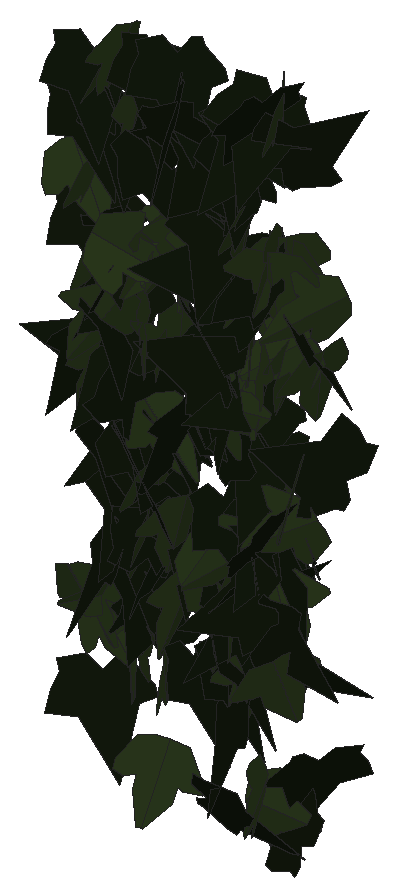
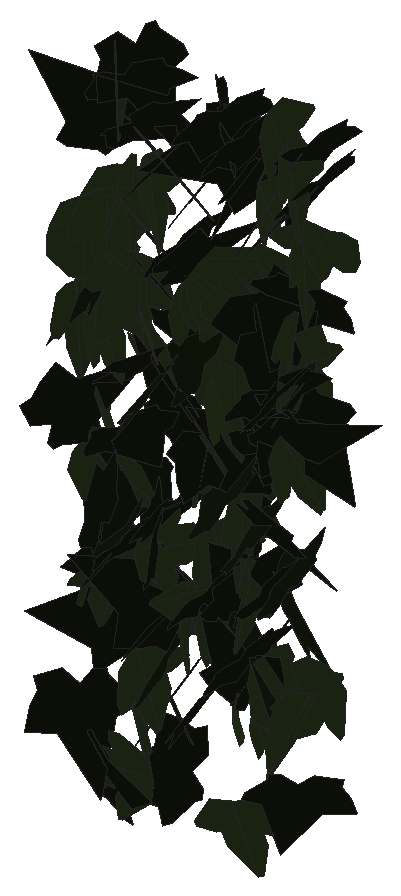
# SketchUp Ruby script. Lengths in inches.
U = 1.inch
M = Sketchup.active_model
def pt(a) = Geom::Point3d.new(a.map { |v| v * U })
def face(e, loops, mat)
  f = e.add_face(loops[0].map { |a| pt(a) })
  loops[1..].each { |l| e.add_face(l.map { |a| pt(a) }).erase! }
  f.material = f.back_material = mat if mat
  f
end
# faces: each face lists its corners as indices into pts; further lists are holes
def faces(e, pts, list, mat = nil) = list.each { |f| face(e, (f[0].is_a?(Array) ? f : [f]).map { |l| l.map { |i| pts[i] } }, mat) }
# xy, xz, yz: faces in a plane at the given z, y or x. An outline is a flat list of corners, or four numbers for a rectangle; further outlines are holes
def ring(l) = l.size == 4 ? [[l[0], l[1]], [l[2], l[1]], [l[2], l[3]], [l[0], l[3]]] : l.each_slice(2).to_a
def flat(e, list, mat, &to3) = list.each { |f| face(e, (f[0].is_a?(Array) ? f : [f]).map { |l| ring(l).map { |u, v| to3.(u, v) } }, mat) }
def xy(e, z, list, mat = nil) = flat(e, list, mat) { |x, y| [x, y, z] }
def xz(e, y, list, mat = nil) = flat(e, list, mat) { |x, z| [x, y, z] }
def yz(e, x, list, mat = nil) = flat(e, list, mat) { |y, z| [x, y, z] }
def lines(e, pts, list) = list.each { |a, b| e.add_line(pt(pts[a]), pt(pts[b])) }
# prism: a flat outline (further loops are holes) pulled along v
def prism(e, loops, v, mat = nil)
  f = face(e, loops, mat); d = Geom::Vector3d.new(v.map { |x| x * U })
  f.pushpull(f.normal.samedirection?(d) ? d.length : -d.length)
end
def box(e, o, s, mat = nil) = prism(e, [[o, [o[0] + s[0], o[1], o[2]], [o[0] + s[0], o[1] + s[1], o[2]], [o[0], o[1] + s[1], o[2]]]], [0, 0, s[2]], mat)
def at(x, y, z, deg = 0) = Geom::Transformation.translation(pt([x, y, z])) * Geom::Transformation.rotation(ORIGIN, Z_AXIS, deg.degrees)
def axes(o, x, y, z) = Geom::Transformation.new([*x, 0, *y, 0, *z, 0, *pt(o).to_a, 1])
def part(name) = M.definitions.add(name)
# library, detail: a bought-in or finely detailed component or shape, given as its bounding box
def library(name, o, s) = part(name).tap { |d| box(d.entities, o, s) }
def detail(e, o, s) = box(e.add_group.entities, o, s)
def put(e, d, t, mat = nil) = e.add_instance(d, t).tap { |i| i.material = mat if mat }
def group(e, t, mat = nil) = e.add_group.tap { |g| g.transformation = t; g.material = mat if mat }.entities
root = M.entities
M.materials.add("efeu1").color = [18, 25, 13]
M.materials.add("efeu2").color = [43, 57, 29]
c1 = part("ivyleaf_9")
p = [[1.54,2.16,1.25],[1.36,2.04,1.19],[-0.21,0.99,0.68],[-0.71,1.11,0.82],[-0.85,0.86,0.67],[-0.8,0.17,0.21],
  [-0.9,-0.01,0.1],[-0.67,-0.16,-0.02],[-0.08,-0.08,-0.05],[-0.03,-0.6,-0.4],[0.65,-0.88,-0.66],[0.83,-0.6,-0.49],
  [1.29,-0.42,-0.43],[1.8125,-0.07,-0.26],[1.21,0.44,0.15]]
faces(c1.entities,p,[[0,1,2,3,4,5,6,7,8,9,10,11,12,13,14]],"efeu1")
c2 = part("ivyleaf_10")
p = [[0,0.5,-0.03],[-0.0625,2.02,-0.43],[-0.19,2.01,-0.46],[-0.54,1.05,-0.29],[-0.52,0.625,-0.18],[-0.83,0.76,-0.28],
  [-1.16,0.64,-0.33],[-1.15,0.33,-0.24],[-0.77,-0.39,0.02],[-0.3,-0.51,0.16],[0.04,-0.48,0.23],[-0.02,2.01,-0.4375],
  [-0.06,2.01,-0.43],[0.04,-0.49,0.23],[0.67,-0.49,0.14],[1.38,0.36,-0.2],[1.375,0.51,-0.24],[0.81,0.65,-0.19],
  [0.62,0.59,-0.15],[0.6,1.09,-0.28],[0.5,1.23,-0.31]]
faces(c2.entities,p,[[0,1,2,3,4,5,6,7,8,9,10],[11,12,0,13,14,15,16,17,18,19,20]],"efeu2")
put(root,c1,axes([31.45,222.08,226.97],[0.14956,-0.33063,0.34397],[-0.15429,0.30759,0.36275],[-0.45147,-0.21465,-0.01002]))
put(root,c2,axes([30.55,222.25,229.83],[-0.21795,-0.34953,0.28342],[-0.15304,-0.23856,-0.4119],[0.42317,-0.2663,-0.00299]))
put(root,c2,axes([33.16,222.05,223.6],[0.30428,-0.36826,-0.14765],[-0.08218,0.12353,-0.47748],[0.38815,0.31484,0.01465]))
put(root,c1,axes([30.61,222.21,226.32],[-0.40272,0.13792,-0.26228],[0.23987,-0.10813,-0.42517],[-0.174,-0.46828,0.02093]))
put(root,c1,axes([31.2,222.05,232.53],[0.22113,-0.38594,-0.22837],[-0.10686,0.20194,-0.44475],[0.43552,0.2455,0.00682]))
put(root,c2,axes([33.5,221.99,225.47],[-0.27696,-0.38547,-0.15717],[0.0796,0.13626,-0.47444],[0.4086,-0.28783,-0.01411]))
put(root,c1,axes([32.36,222.05,223.1],[0.41261,-0.11866,0.25626],[0.24759,-0.06623,-0.42932],[0.13583,0.48118,0.0041]))
put(root,c1,axes([31.6,222.28,233.29],[-0.27418,0.11213,-0.4028],[0.37252,-0.15324,-0.29623],[-0.18989,-0.46254,0.00049]))
put(root,c1,axes([32.27,222.45,230.77],[-0.2241,-0.0434,0.44485],[-0.31262,-0.34045,-0.1907],[0.31945,-0.36361,0.12545]))
put(root,c1,axes([32.58,222.27,224.45],[-0.35983,0.05267,-0.34314],[0.33766,-0.06174,-0.36356],[-0.08067,-0.49337,0.00886]))
put(root,c1,axes([33.2,222.12,226],[0.04453,-0.04723,-0.49577],[0.44248,0.23216,0.01763],[0.22853,-0.44031,0.06247]))
put(root,c1,axes([33.13,222.16,226.34],[-0.44882,0.14556,0.16544],[-0.15751,0.0506,-0.47184],[-0.15411,-0.47566,0.00043]))
put(root,c2,axes([33.35,222.09,231.46],[-0.4619,-0.19142,0.00291],[-0.00274,-0.00098,-0.49999],[0.19142,-0.46191,-0.00014]))
put(root,c2,axes([33.2,222.41,231.48],[-0.02504,0.27389,-0.41756],[0.01105,-0.41768,-0.27463],[-0.49925,-0.02298,0.01487]))
put(root,c2,axes([32.4,222.28,228.9375],[0.08497,-0.1088,-0.48056],[0.42623,-0.22842,0.12708],[-0.24719,-0.43126,0.05394]))
put(root,c2,axes([30.66,222,230.87],[0.15039,0.11673,0.46234],[0.379,0.26494,-0.19017],[-0.28938,0.40766,-0.00879]))
put(root,c1,axes([30.03,222.28,232.76],[0.13252,-0.47272,-0.09475],[0.0012,0.09859,-0.49018],[0.48212,0.12969,0.02727]))
put(root,c1,axes([32.46,222.14,229.5],[-0.27431,0.13469,0.39574],[-0.35996,0.16457,-0.30552],[-0.21256,-0.45252,0.00668]))
put(root,c1,axes([33.19,222.24,231.21],[-0.45908,0.1956,0.03148],[-0.02973,0.01054,-0.499],[-0.19587,-0.46003,0.00195]))
put(root,c1,axes([32.82,222.29,226.01],[-0.46992,0.15477,-0.07226],[0.06609,-0.03029,-0.49469],[-0.1575,-0.47448,0.00801]))
put(root,c1,axes([32.34,222.21,228.26],[-0.20283,0.17516,0.42211],[0.29655,-0.30094,0.26738],[0.34773,0.35882,0.01819]))
put(root,c2,axes([31.2,222.49,224.57],[-0.00541,0.02291,0.49945],[0.40198,-0.2968,0.01797],[0.29729,0.40173,-0.01521]))
put(root,c2,axes([31.6,222.45,225.875],[0.02998,-0.44579,0.22443],[0.05607,-0.2204,-0.44528],[0.49594,0.05187,0.03677]))
put(root,c1,axes([33.21,221.85,227.34],[0.10913,0.42255,0.24402],[0.06265,0.23584,-0.43641],[-0.48391,0.12583,-0.00147]))
put(root,c1,axes([30.0625,222.44,233.33],[-0.02975,-0.49473,-0.06601],[0.01847,0.065,-0.49541],[0.49877,-0.03191,0.01441]))
put(root,c1,axes([33.04,222.25,233.67],[-0.06447,0.41498,-0.27135],[0.03559,-0.26906,-0.41993],[-0.49455,-0.07346,0.00515]))
put(root,c2,axes([32.45,222.63,226.62],[-0.00025,-0.09169,0.49152],[-0.02745,-0.49078,-0.09157],[0.49925,-0.02703,-0.00479]))
put(root,c2,axes([32.75,222.39,229.68],[0.41358,-0.14747,0.23918],[0.22269,-0.08751,-0.43903],[0.17135,0.46967,-0.0067]))
put(root,c1,axes([30.79,222.63,225.39],[0.01053,-0.37536,0.33014],[0.02863,-0.32922,-0.37523],[0.49907,0.0268,0.01456]))
put(root,c1,axes([30.29,222.55,229.55],[0.12032,-0.43719,0.21068],[0.06195,-0.20145,-0.45341],[0.48134,0.13521,0.00569]))
put(root,c1,axes([30.26,222.39,229.23],[0.02593,0.28829,-0.40769],[-0.01629,-0.40754,-0.28922],[-0.49906,0.02828,-0.01174]))
put(root,c2,axes([30.79,222.53,229.62],[-0.15141,0.16736,-0.44617],[0.2085,-0.39769,-0.21993],[-0.42849,-0.25265,0.05064]))
put(root,c2,axes([33.87,222.61,230.84],[-0.0705,-0.18459,0.4593],[-0.16812,-0.42743,-0.19758],[0.46558,-0.18229,-0.0018]))
put(root,c2,axes([33.46,222.42,228.25],[0.31377,-0.37857,0.0907],[0.05557,-0.07174,-0.4917],[0.3853,0.31864,-0.00294]))
put(root,c2,axes([33.59,222.43,227.5],[-0.22618,-0.11469,0.43092],[-0.36823,-0.22448,-0.25302],[0.25151,-0.4318,0.01708]))
put(root,c2,axes([29.97,222.23,231.87],[0.37134,0.27532,0.19055],[0.15152,0.11557,-0.46226],[-0.29858,0.40105,0.0024]))
put(root,c1,axes([31.72,222.49,228.49],[-0.10576,0.25807,-0.41499],[0.12603,-0.39583,-0.27827],[-0.47216,-0.16346,0.01867]))
put(root,c2,axes([32.36,222.31,225.8],[0.38459,-0.30392,-0.0986],[-0.04094,0.10615,-0.48688],[0.31688,0.38258,0.05677]))
put(root,c2,axes([31.21,222.35,228.36],[-0.39728,-0.12288,-0.27761],[0.30065,-0.09576,-0.38786],[0.04216,-0.47511,0.14998]))
put(root,c1,axes([33,222.69,229.1],[-0.35126,-0.14312,0.32577],[-0.18958,-0.31212,-0.34153],[0.30112,-0.36346,0.165]))
put(root,c2,axes([32.72,222.34,231.95],[0.11405,-0.47814,-0.09149],[-0.01916,0.08949,-0.49155],[0.48644,0.11563,0.00209]))
put(root,c1,axes([30.14,222.45,231.15],[-0.21262,-0.28904,-0.34821],[0.29254,0.20574,-0.34941],[0.34527,-0.35231,0.08163]))
put(root,c1,axes([31.74,222.76,232.1],[-0.10251,-0.31373,0.37559],[-0.00552,-0.38298,-0.3214],[0.48935,-0.07004,0.07506]))
put(root,c1,axes([32,222.69,231.32],[-0.07971,-0.47321,0.14042],[0.0014,-0.14246,-0.47927],[0.4936,-0.07601,0.02403]))
put(root,c1,axes([32.88,222.28,232.4],[-0.35996,0.28801,0.19359],[-0.16122,0.10821,-0.46076],[-0.3073,-0.39413,0.01497]))
put(root,c1,axes([31.31,222.1,232.77],[0.0628,0.1577,-0.47031],[0.20494,0.42346,0.16936],[0.45173,-0.21404,-0.01145]))
put(root,c1,axes([32.9,222.625,233.47],[-0.29716,-0.39646,-0.06717],[0.03296,0.05923,-0.49538],[0.40076,-0.29884,-0.00906]))
put(root,c2,axes([30.15,222.37,231.75],[0.06623,-0.48218,-0.11454],[0.01015,0.11686,-0.48605],[0.49549,0.06206,0.02527]))
put(root,c1,axes([30.82,222.19,228.27],[-0.03168,-0.05473,0.49599],[0.47762,0.14058,0.04602],[-0.14449,0.4767,0.04337]))
put(root,c2,axes([33.4375,222.53,230.1],[-0.30616,0.01098,0.39515],[-0.35543,-0.22639,-0.2691],[0.17301,-0.44568,0.14642]))
put(root,c1,axes([30.55,222.79,226.68],[-0.10428,-0.42688,0.23853],[-0.03437,-0.23689,-0.43898],[0.48779,-0.10795,0.02006]))
put(root,c1,axes([32.67,222.77,232.92],[-0.29058,-0.37259,0.16354],[-0.06611,-0.15506,-0.47073],[0.40149,-0.29519,0.04085]))
put(root,c2,axes([31.5,222.5,226.99],[-0.07434,-0.49198,0.04925],[-0.00015,-0.04978,-0.49752],[0.49444,-0.07398,0.00725]))
put(root,c1,axes([32.29,222.75,232.42],[0.01345,-0.46907,0.1726],[0.04795,-0.17065,-0.46752],[0.49751,0.02913,0.04039]))
put(root,c2,axes([30.18,222.63,228.86],[-0.00834,-0.46213,0.19071],[-0.01572,-0.1904,-0.46206],[0.49968,-0.01371,-0.01135]))
put(root,c2,axes([29.87,222.41,225.39],[-0.44855,0.07356,-0.2083],[0.20392,-0.04343,-0.45446],[-0.08495,-0.49265,0.00896]))
put(root,c2,axes([32.87,222.5,223.0625],[-0.0275,0.0027,-0.49924],[0.47636,-0.14949,-0.02705],[-0.14941,-0.47712,0.00565]))
put(root,c1,axes([30.6,222.73,229.05],[-0.38326,-0.31425,0.06602],[-0.04363,-0.05088,-0.49549],[0.31813,-0.38556,0.01157]))
put(root,c2,axes([30.48,222.74,224.45],[-0.10948,0.1082,-0.47572],[0.20763,-0.43086,-0.14578],[-0.44148,-0.22947,0.04941]))
put(root,c2,axes([31.42,222.51,229.28],[-0.48567,-0.07669,0.09078],[0.0906,0.00822,0.49166],[-0.0769,0.49401,0.00591]))
put(root,c1,axes([30.42,222.71,228.82],[-0.25914,-0.27677,-0.32595],[-0.10576,-0.32781,0.36243],[-0.41432,0.25679,0.11135]))
put(root,c2,axes([30.4,222.64,233.57],[0.05833,-0.46831,0.16518],[0.04309,-0.16092,-0.47143],[0.49471,0.06923,0.02158]))
put(root,c1,axes([32.22,222.5,227.33],[0.14804,-0.43981,-0.18615],[-0.05579,0.17763,-0.46404],[0.47431,0.15816,0.00352]))
put(root,c1,axes([32.78,222.49,230.62],[-0.44872,0.20334,0.08543],[-0.08032,0.02972,-0.49261],[-0.20541,-0.45582,0.006]))
put(root,c1,axes([30.65,222.7,230.46],[-0.24181,0.17685,-0.40032],[0.2012,-0.36123,-0.28112],[-0.38865,-0.29704,0.10353]))
put(root,c2,axes([30.46,222.77,225.25],[-0.10266,0.07177,-0.48405],[-0.34574,-0.36066,0.01985],[-0.3463,0.33879,0.12368]))
put(root,c2,axes([31.14,222.53,223.11],[0.47326,0.13712,-0.08501],[-0.08148,-0.02425,-0.49272],[-0.13925,0.48022,-0.00061]))
put(root,c1,axes([30.28,222.78,232.26],[0.02946,-0.46755,0.17473],[0.07932,-0.16842,-0.46405],[0.49279,0.05506,0.06425]))
put(root,c1,axes([30.75,222.85,227.36],[-0.03931,-0.34855,0.35633],[0.10717,-0.35499,-0.33541],[0.48679,0.05001,0.10262]))
put(root,c2,axes([31.19,222.66,230.87],[0.14994,0.34992,-0.32415],[-0.23739,-0.23998,-0.36886],[-0.41372,0.26451,0.09417]))
put(root,c2,axes([31.13,222.4,227.52],[-0.01285,-0.46823,-0.17493],[0.00423,0.17488,-0.4684],[0.49982,-0.01352,-0.00053]))
put(root,c2,axes([31.42,222.73,231.04],[-0.06118,-0.40717,0.28367],[-0.04991,-0.27932,-0.41169],[0.49373,-0.07869,-0.00646]))
put(root,c1,axes([31.65,222.59,224.7],[0.20641,-0.4494,-0.07372],[-0.0324,0.06625,-0.49453],[0.45425,0.20893,-0.00177]))
put(root,c1,axes([32.25,222.63,225.06],[0.28933,-0.40221,0.06718],[0.03319,-0.05887,-0.49541],[0.40643,0.29113,-0.00737]))
put(root,c1,axes([32.85,222.77,228.34],[-0.24012,-0.43855,0.00437],[-0.00165,-0.00408,-0.49998],[0.43857,-0.24013,0.00051]))
put(root,c1,axes([32.04,222.72,229.22],[-0.26305,-0.13734,-0.40242],[0.4215,-0.02182,-0.26807],[0.05608,-0.48027,0.12726]))
put(root,c2,axes([30.51,222.76,232.61],[0.13595,-0.38936,0.2827],[0.19033,-0.2263,-0.40319],[0.44192,0.21724,0.08668]))
put(root,c1,axes([33.05,222.47,225.3],[0.34838,-0.08407,0.34866],[0.34021,-0.07643,-0.35835],[0.11355,0.48692,0.00395]))
put(root,c1,axes([31.02,222.22,225.61],[-0.10117,0.39647,0.28736],[-0.10067,0.27031,-0.40841],[-0.4792,-0.1405,0.02513]))
put(root,c1,axes([33.82,222.46,224],[0.08257,0.43198,-0.23786],[-0.04008,-0.23449,-0.43978],[-0.4915,0.0917,-0.0041]))
put(root,c2,axes([30.58,222.7,224.61],[-0.2832,0.08256,0.40371],[0.3731,-0.15657,0.29374],[0.17492,0.46762,0.02707]))
put(root,c1,axes([31.55,222.77,229.76],[0.23569,-0.34482,0.27487],[0.14564,-0.2333,-0.41756],[0.41622,0.27689,-0.00953]))
put(root,c1,axes([31.1,222.32,226.25],[-0.19769,-0.14847,0.4346],[0.33252,0.28009,0.24694],[-0.31678,0.38666,-0.012]))
put(root,c1,axes([33.9,222.85,228.12],[-0.02076,-0.02498,0.49894],[-0.43456,-0.24543,-0.03037],[0.24643,-0.4349,-0.01152]))
put(root,c1,axes([33.56,222.36,222.77],[-0.12622,0.14516,0.46152],[-0.29871,0.35182,-0.19235],[-0.38058,-0.32427,-0.00209]))
put(root,c2,axes([32.46,222.8,230.16],[0.24736,-0.25954,0.3485],[0.26713,-0.22546,-0.35751],[0.34272,0.36306,0.02712]))
put(root,c1,axes([30.85,222.79,233.35],[0.00947,-0.49988,0.00536],[-0.00413,-0.00544,-0.49995],[0.49989,0.00943,-0.00423]))
put(root,c2,axes([30.21,222.45,230.53],[-0.01989,-0.44762,-0.2219],[0.07256,0.21713,-0.44451],[0.49431,-0.04988,0.05632]))
put(root,c1,axes([32.27,222.8125,227],[0.10574,-0.0619,-0.48475],[0.47247,-0.11378,0.11759],[-0.12487,-0.48293,0.03443]))
put(root,c1,axes([30.0625,222.65,223.93],[-0.19938,-0.36217,-0.28122],[0.13634,0.24596,-0.41342],[0.43779,-0.24153,0.00068]))
put(root,c2,axes([31.4,222.86,231.01],[-0.23573,-0.25634,0.35877],[-0.08485,-0.37285,-0.32215],[0.4327,-0.21276,0.13229]))
put(root,c2,axes([31.79,222.38,228.55],[-0.33125,0.27572,0.25347],[-0.18597,0.17263,-0.43083],[-0.32509,-0.3797,-0.01182]))
put(root,c2,axes([30.2,222.59,233.1],[0.09488,-0.48368,-0.08398],[-0.01716,0.08221,-0.4929],[0.49062,0.09641,-0.001]))
put(root,c1,axes([30.33,222.5,230.52],[0.23388,-0.02882,0.44099],[0.43892,-0.04297,-0.23559],[0.05148,0.49732,0.0052]))
put(root,c1,axes([33.36,222.55,230.46],[0.41065,-0.24584,-0.14468],[-0.12491,0.07302,-0.47861],[0.25645,0.42922,-0.00145]))
put(root,c1,axes([31.24,222.74,233.55],[-0.02107,-0.47641,-0.15029],[0.0162,0.14969,-0.47679],[0.49929,-0.02496,0.00913]))
put(root,c2,axes([33.17,222.62,231.41],[-0.3308,-0.3748,-0.00984],[0.00698,0.00696,-0.4999],[0.37486,-0.33087,0.00063]))
put(root,c2,axes([33.1,222.54,233.59],[0.19002,-0.41882,-0.19616],[-0.02562,0.20222,-0.45657],[0.46178,0.18356,0.05539]))
put(root,c2,axes([30.99,222.41,226.59],[0.06227,-0.33775,-0.36338],[-0.02822,0.36323,-0.34244],[0.4953,0.06316,0.02618]))
put(root,c1,axes([30.7,222.74,227.79],[-0.48955,0.08952,0.04825],[-0.04901,0.00019,-0.49759],[-0.08911,-0.49192,0.00859]))
put(root,c1,axes([29.95,222.97,227.09],[0.05422,-0.38349,0.31622],[0.12464,-0.29744,-0.38209],[0.48117,0.12026,0.06334]))
put(root,c1,axes([30.9,222.6,225.04],[-0.25961,0.09423,0.4168],[0.36163,-0.21136,0.27304],[0.22765,0.44322,0.04159]))
put(root,c2,axes([33.7,222.65,229.875],[-0.07785,-0.49111,-0.05247],[0.00777,0.05189,-0.49724],[0.49384,-0.07824,-0.00044]))
put(root,c2,axes([32.51,222.8,224.93],[-0.07748,-0.47708,0.12804],[0.05021,-0.13654,-0.47837],[0.4914,-0.06127,0.06907]))
put(root,c2,axes([33.2,222.8125,229.87],[0.08744,-0.47597,0.12574],[0.0247,-0.1233,-0.48393],[0.49167,0.09084,0.00195]))
put(root,c1,axes([31.04,222.95,227.93],[0.10855,-0.4114,0.26262],[0.14579,-0.22942,-0.41966],[0.46579,0.16769,0.07015]))
put(root,c1,axes([30.24,223.09,229.68],[-0.16779,-0.3074,0.35686],[-0.05409,-0.36375,-0.33876],[0.46789,-0.15229,0.08882]))
put(root,c2,axes([33.08,222.58,226.18],[0.13076,0.47606,0.07917],[0.0238,0.07557,-0.49368],[-0.48201,0.13287,-0.0029]))
put(root,c1,axes([32.63,223.06,226.86],[-0.14737,-0.42763,0.2131],[-0.01471,-0.21884,-0.44932],[0.47756,-0.1387,0.05192]))
put(root,c2,axes([31.57,222.98,230.83],[-0.0916,-0.36554,0.32861],[0.11662,-0.34089,-0.34669],[0.4775,0.01313,0.14771]))
put(root,c2,axes([31.2,222.83,229.41],[0.09559,-0.47624,0.11858],[0.02115,-0.11669,-0.48573],[0.49032,0.09788,-0.00216]))
put(root,c1,axes([33.16,222.58,232.68],[-0.04191,-0.07965,0.49183],[0.49813,0.00344,0.04301],[-0.01024,0.4936,0.07906]))
put(root,c1,axes([32.12,222.92,225.85],[0.10769,-0.48489,0.05731],[0.00956,-0.05658,-0.4967],[0.48817,0.10808,-0.00292]))
put(root,c1,axes([32.85,222.94,226.7],[0.17529,-0.43832,0.16478],[0.06233,-0.15254,-0.47206],[0.4641,0.18604,0.00117]))
put(root,c2,axes([32.83,222.6,230.57],[-0.31217,-0.32535,-0.21608],[0.17338,0.13243,-0.44989],[0.34998,-0.35582,0.03014]))
put(root,c1,axes([32.43,222.44,225.75],[0.17309,0.43125,-0.18456],[0.0379,0.18322,0.46367],[0.46755,-0.17451,0.03073]))
put(root,c1,axes([33.03,223.02,227.04],[0.09169,-0.19115,0.45283],[0.16613,-0.42148,-0.21155],[0.46259,0.18925,-0.01378]))
put(root,c1,axes([30.29,222.93,229.86],[-0.11186,-0.48353,-0.06072],[0.01845,0.05806,-0.49628],[0.48698,-0.11326,0.00485]))
put(root,c1,axes([30.75,222.88,231.87],[0.06066,-0.48172,0.11943],[0.01049,0.12154,0.48489],[-0.4962,-0.05632,0.02485]))
put(root,c2,axes([30.11,222.54,225.05],[0.05164,0.4609,0.18683],[0.02344,0.18537,-0.46378],[-0.49677,0.05665,-0.00246]))
put(root,c1,axes([31.95,222.8,224.76],[0.25786,-0.42138,-0.07713],[-0.04192,0.06477,-0.49401],[0.42632,0.26124,-0.00193]))
put(root,c1,axes([31.28,223.01,226.55],[-0.01449,-0.49427,0.07407],[0.0106,-0.07439,-0.49432],[0.49968,-0.01275,0.01263]))
put(root,c2,axes([33.13,222.71,231.3],[-0.45849,0.1605,-0.11843],[0.10505,-0.05808,-0.48538],[-0.16956,-0.46997,0.01953]))
put(root,c2,axes([31.82,222.36,226.1],[0.09024,0.08243,-0.48483],[0.16028,0.46108,0.10822],[0.46494,-0.17495,0.05679]))
put(root,c1,axes([32.31,222.92,229.1],[0.21257,-0.44915,0.05546],[0.02085,-0.05149,-0.4969],[0.45208,0.21357,-0.00316]))
put(root,c1,axes([30.68,223.05,225.79],[-0.04725,-0.48735,0.10126],[-0.00422,-0.10132,-0.48961],[0.49774,-0.04712,0.00546]))
